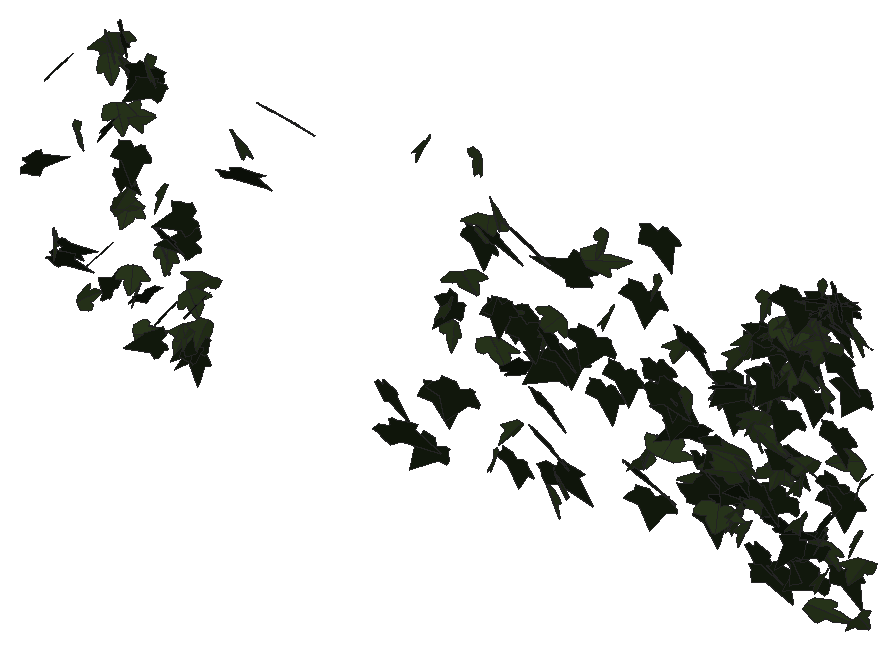
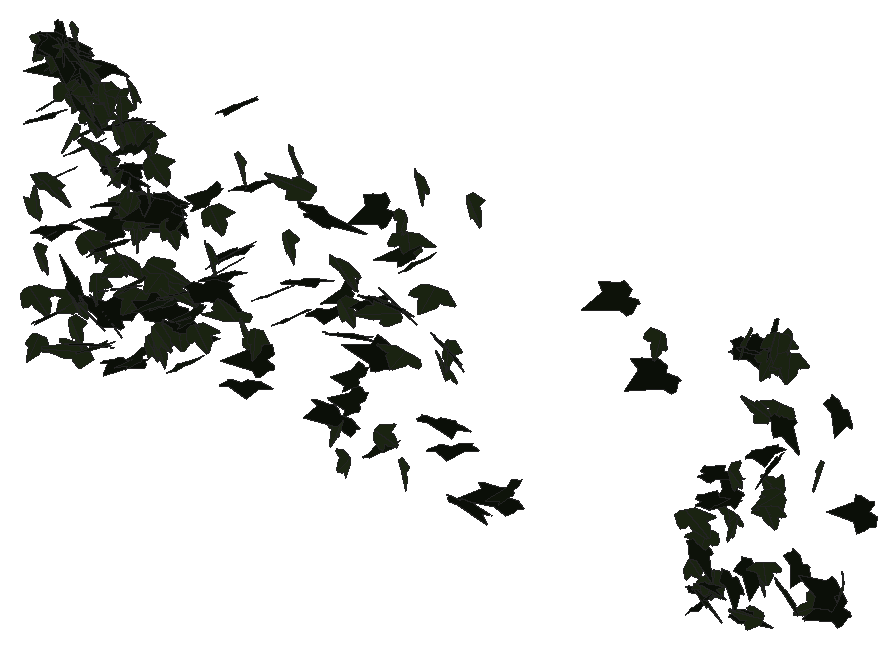
# SketchUp Ruby script. Lengths in millimetres.
U = 1.mm
M = Sketchup.active_model
def pt(a) = Geom::Point3d.new(a.map { |v| v * U })
def face(e, loops, mat)
  f = e.add_face(loops[0].map { |a| pt(a) })
  loops[1..].each { |l| e.add_face(l.map { |a| pt(a) }).erase! }
  f.material = f.back_material = mat if mat
  f
end
# faces: each face lists its corners as indices into pts; further lists are holes
def faces(e, pts, list, mat = nil) = list.each { |f| face(e, (f[0].is_a?(Array) ? f : [f]).map { |l| l.map { |i| pts[i] } }, mat) }
# xy, xz, yz: faces in a plane at the given z, y or x. An outline is a flat list of corners, or four numbers for a rectangle; further outlines are holes
def ring(l) = l.size == 4 ? [[l[0], l[1]], [l[2], l[1]], [l[2], l[3]], [l[0], l[3]]] : l.each_slice(2).to_a
def flat(e, list, mat, &to3) = list.each { |f| face(e, (f[0].is_a?(Array) ? f : [f]).map { |l| ring(l).map { |u, v| to3.(u, v) } }, mat) }
def xy(e, z, list, mat = nil) = flat(e, list, mat) { |x, y| [x, y, z] }
def xz(e, y, list, mat = nil) = flat(e, list, mat) { |x, z| [x, y, z] }
def yz(e, x, list, mat = nil) = flat(e, list, mat) { |y, z| [x, y, z] }
def lines(e, pts, list) = list.each { |a, b| e.add_line(pt(pts[a]), pt(pts[b])) }
# prism: a flat outline (further loops are holes) pulled along v
def prism(e, loops, v, mat = nil)
  f = face(e, loops, mat); d = Geom::Vector3d.new(v.map { |x| x * U })
  f.pushpull(f.normal.samedirection?(d) ? d.length : -d.length)
end
def box(e, o, s, mat = nil) = prism(e, [[o, [o[0] + s[0], o[1], o[2]], [o[0] + s[0], o[1] + s[1], o[2]], [o[0], o[1] + s[1], o[2]]]], [0, 0, s[2]], mat)
def at(x, y, z, deg = 0) = Geom::Transformation.translation(pt([x, y, z])) * Geom::Transformation.rotation(ORIGIN, Z_AXIS, deg.degrees)
def axes(o, x, y, z) = Geom::Transformation.new([*x, 0, *y, 0, *z, 0, *pt(o).to_a, 1])
def part(name) = M.definitions.add(name)
# library, detail: a bought-in or finely detailed component or shape, given as its bounding box
def library(name, o, s) = part(name).tap { |d| box(d.entities, o, s) }
def detail(e, o, s) = box(e.add_group.entities, o, s)
def put(e, d, t, mat = nil) = e.add_instance(d, t).tap { |i| i.material = mat if mat }
def group(e, t, mat = nil) = e.add_group.tap { |g| g.transformation = t; g.material = mat if mat }.entities
root = M.entities
M.materials.add("efeu1").color = [18, 25, 13]
M.materials.add("efeu2").color = [43, 57, 29]
c1 = part("ivyleaf_9")
p = [[39.1,54.8,31.7],[34.5,51.8,30.2],[-5.3,25.2,17.3],[-17.9,28.3,20.9],[-21.6,21.7,17],[-20.2,4.3,5.3],
  [-22.9,-0.3,2.5],[-17.1,-4,-0.6],[-2,-2.1,-1.2],[-0.7,-15.4,-10.1],[16.6,-22.3,-16.7],[21.1,-15.1,-12.5],
  [32.7,-10.7,-11],[46.1,-1.8,-6.6],[30.8,11.2,3.8]]
faces(c1.entities,p,[[0,1,2,3,4,5,6,7,8,9,10,11,12,13,14]],"efeu1")
c2 = part("ivyleaf_10")
p = [[0,12.8,-0.8],[-1.5,51.3,-10.9],[-4.9,51,-11.6],[-13.6,26.5,-7.3],[-13.2,15.9,-4.6],[-21.1,19.3,-7.2],
  [-29.5,16.3,-8.3],[-29.2,8.3,-6.2],[-19.7,-9.8,0.5],[-7.6,-13,4],[1,-12.2,5.8],[-0.4,51.1,-11.1],
  [-1.5,51.1,-10.9],[1,-12.4,5.9],[16.9,-12.4,3.5],[35.1,9.1,-5.1],[35,12.9,-6.1],[20.5,16.4,-4.9],
  [15.8,15,-3.8],[15.3,27.6,-7.1],[12.8,31.3,-7.8]]
faces(c2.entities,p,[[0,1,2,3,4,5,6,7,8,9,10],[11,12,0,13,14,15,16,17,18,19,20]],"efeu2")
put(root,c1,axes([356.5,756.3,2993.2],[0.34233,0.69768,-0.91695],[0.14407,0.92137,0.73718],[1.39828,-0.26574,0.14853]))
put(root,c1,axes([418.9,777,3252.7],[0.1319,0.98378,0.6336],[-0.03652,0.63842,-0.98615],[-1.42713,0.07459,0.08379]))
put(root,c2,axes([403.1,793,2800.9],[-0.36307,0.76759,-0.76025],[0.21719,-0.74294,-0.8198],[-1.30002,-0.3385,0.07536]))
put(root,c1,axes([401.6,799.6,2740.1],[1.21232,0.1716,0.53653],[0.65202,0.05658,-1.00794],[-0.21716,1.12788,-0.03107]))
put(root,c1,axes([421.4,807.3,2769.8],[0.95036,0.3908,-0.68763],[0.74884,0.30998,0.87151],[0.60854,-0.99175,0.00144]))
put(root,c2,axes([458.5,805,3095.3],[-0.68531,0.96396,0.23463],[-0.13774,0.20577,-1.11567],[-1.20251,-0.57293,-0.00592]))
put(root,c2,axes([517.1,757,2684.8],[0.04475,-0.10133,1.11114],[-0.06553,1.11029,0.10303],[-1.35963,-0.05685,0.0316]))
put(root,c1,axes([541.4,772.1,2796.8],[0.26817,0.86274,0.67767],[0.00973,0.68986,-0.88085],[-1.33838,0.17788,0.12938]))
put(root,c2,axes([547.8,807.2,3356.1],[-1.01402,-0.78103,-0.11814],[0.07767,0.1047,-1.14008],[0.96056,-0.83297,-0.03253]))
put(root,c1,axes([578.3,789.1,2721.7],[-0.43352,0.78424,0.68069],[-0.43135,0.58508,-0.85866],[-1.19121,-0.49727,0.06321]))
put(root,c1,axes([585.2,789.4,3174],[-0.53232,0.98978,-0.4697],[0.20509,-0.43911,-1.08148],[-1.32078,-0.4671,0.02137]))
put(root,c2,axes([571.2,780.6,3389.5],[-0.88104,0.89475,-0.19022],[0.1387,-0.15268,-1.1498],[-1.10734,-0.73102,0.00732]))
put(root,c2,axes([569.7,785.1,3330.9],[0.51505,1.08872,0.04324],[0.02313,0.03903,-1.1677],[-1.32908,0.42258,-0.00356]))
put(root,c2,axes([585.9,802,3391.7],[-1.06774,-0.75615,-0.11022],[0.10725,0.06683,-1.15658],[0.92606,-0.87957,0.00687]))
put(root,c1,axes([607.2,784.1,3414],[0.6622,-0.12279,-1.03457],[-1.13242,0.47276,-0.5431],[0.5772,1.06839,0.12142]))
put(root,c2,axes([590.6,788.3,3204.1],[1.27648,0.36666,0.39342],[0.45387,0.128,-1.10868],[-0.47379,1.11046,-0.00211]))
put(root,c2,axes([603.4,815.8,2937.4],[1.23029,0.3806,-0.17497],[-0.19692,-0.06786,-1.07785],[-0.4716,1.02125,-0.00641]))
put(root,c2,axes([602.9,788.6,2962.1],[-0.45813,-0.38786,-0.98717],[0.83705,0.70976,-0.53986],[0.98676,-0.78215,-0.00037]))
put(root,c1,axes([608.7,781.9,3053.1],[0.68449,-0.6018,-0.76512],[-0.51748,0.64372,-0.81735],[1.06892,0.697,0.09426]))
put(root,c2,axes([612.2,777.4,2965.3],[-0.0764,-1.05409,0.53907],[0.03605,0.53827,1.05595],[-1.44396,0.06921,-0.00216]))
put(root,c2,axes([615.8,796.3,3326.9],[-1.3192,0.40401,-0.15754],[0.19032,-0.03247,-1.15407],[-0.49362,-1.09224,-0.02396]))
put(root,c1,axes([616.8,819.6,3093.1],[-0.47829,-1.05459,-0.21128],[0.08194,0.20043,-1.12508],[1.30961,-0.39769,-0.00677]))
put(root,c2,axes([622.4,804.9,2775.9],[1.06437,0.63682,-0.05341],[-0.04737,-0.03739,-1.08011],[-0.77821,0.87327,-0.0073]))
put(root,c2,axes([646.2,797.6,2743.1],[0.62335,-0.92071,-0.02251],[-0.00867,0.0218,-1.05298],[1.12357,0.51097,0.00436]))
put(root,c2,axes([618.7,815,3187.5],[0.42237,-0.21402,-1.07935],[1.26282,-0.32055,0.39557],[-0.45546,-1.08725,0.09584]))
put(root,c1,axes([682.3,786.3,3343.4],[0.44286,0.56089,-0.98218],[-0.69273,-0.80175,-0.6677],[-1.1934,0.67353,0.02311]))
put(root,c1,axes([675,781,2745.6],[0.29378,1.04941,0.05142],[0.0185,0.04928,-1.07668],[-1.28169,0.24125,-0.00375]))
put(root,c2,axes([654.6,798,2626.2],[0.2891,-0.01851,-1.04724],[1.22337,0.31416,0.22135],[0.36911,-1.02673,0.08661]))
put(root,c1,axes([704.7,805.7,2618.9],[-1.07946,-0.09292,0.56212],[-0.67914,-0.08022,-0.88948],[0.14809,-1.04519,0.01829]))
put(root,c1,axes([703.3,793.1,3312.8],[-1.34136,-0.29734,0.28822],[-0.32088,-0.13016,-1.13763],[0.39021,-1.12914,0.05524]))
put(root,c2,axes([688.7,784.5,3359.6],[-0.54799,1.07798,0.22484],[-0.07593,0.21758,-1.16754],[-1.34129,-0.45273,-0.02577]))
put(root,c2,axes([698.7,829.5,3008.7],[0.37157,-0.90811,0.59404],[0.23973,-0.56064,-0.9578],[1.30199,0.36239,0.00682]))
put(root,c1,axes([727.6,796.1,2699.6],[-0.19934,1.01209,0.32974],[-0.0478,0.32766,-1.02511],[-1.29775,-0.16753,-0.01289]))
put(root,c2,axes([714,805.4,2861.3],[-0.84808,0.83202,-0.14465],[0.10722,-0.11506,-1.08418],[-1.0247,-0.70066,0.00627]))
put(root,c2,axes([734.8,794.1,2873.1],[1.29469,-0.21206,0.17514],[0.21265,-0.02144,-1.08213],[0.25955,1.07536,0.01296]))
put(root,c1,axes([730.2,778.9,2929.1],[1.31564,-0.24368,-0.01207],[-0.01369,0.0051,-1.10558],[0.29734,1.07845,0.0025]))
put(root,c1,axes([786.5,815.6,2971.5],[-0.95963,-0.32714,0.70864],[-0.78504,-0.29759,-0.85163],[0.53891,-1.01603,0.02127]))
put(root,c1,axes([788.6,826.3,2901.2],[-0.81032,-0.21197,0.84357],[-0.92564,-0.3778,-0.69232],[0.51888,-1.00501,0.08234]))
put(root,c2,axes([790.9,798.5,2678.7],[-0.45719,-0.93259,0.60477],[0.00861,-0.6402,-0.98286],[1.35603,-0.31036,0.21014]))
put(root,c2,axes([793,801.8,2682.6],[0.4401,1.09946,-0.18153],[-0.26091,-0.11895,-1.14543],[-1.33423,0.38592,0.16411]))
put(root,c1,axes([810.8,817.9,2661.6],[-1.14636,-0.56298,0.2136],[-0.18719,-0.15895,-1.09393],[0.71036,-0.95041,0.05643]))
put(root,c1,axes([818.4,807,2641.9],[-1.1866,0.57833,-0.25387],[0.25064,-0.15111,-1.13131],[-0.72864,-0.99379,0.02428]))
put(root,c1,axes([820.4,803.7,2760],[-0.47716,1.05139,-0.17096],[0.07305,-0.16014,-1.12178],[-1.29749,-0.39567,-0.00028]))
put(root,c1,axes([805.4,816.6,2620.4],[0.02539,-1.10274,0.10467],[0.00627,-0.10459,-1.10293],[1.35137,0.0212,0.00315]))
put(root,c2,axes([811.1,787.8,2784.9],[0.86052,0.84982,0.3555],[0.0653,0.40917,-1.08434],[-1.12194,0.67562,0.20955]))
put(root,c2,axes([844.5,806.5,2834.1],[-1.20026,-0.63198,0.5214],[-0.66958,-0.38533,-0.89259],[1.40821,-0.72187,0.01999]))
put(root,c2,axes([838.4,805.2,2707.8],[-0.32691,-0.91343,0.63261],[0.28616,-0.68259,-0.88624],[1.325,-0.07794,0.34748]))
put(root,c2,axes([962.7,777.8,3256.1],[-1.52598,0.70772,0.23513],[-0.36821,0.13602,-1.06916],[-1.37073,-0.82442,0.02544]))
put(root,c1,axes([944.5,778.5,3165.3],[1.81078,0.43116,0.29051],[0.51701,0.10427,-1.04445],[-0.84366,0.98932,-0.01653]))
put(root,c1,axes([1035,805.7,3350.7],[2.10136,-0.17355,0.00871],[0.09052,0.24793,-1.08883],[0.31808,1.07596,0.2523]))
put(root,c1,axes([1364.1,818,2723.6],[1.02261,-0.91059,-0.11841],[-0.13079,0.09693,-1.05725],[1.74271,0.5416,-0.00987]))
put(root,c1,axes([1427.6,766.8,2662.3],[0.19495,-0.10547,-1.05394],[1.20963,0.85316,-0.02361],[1.61262,-0.62721,0.14512]))
put(root,c2,axes([1501.6,796.5,3433.2],[0.20888,-1.12799,0.06776],[0.00593,-0.06778,-1.13331],[2.15064,0.10974,-0.00345]))
put(root,c1,axes([1526.5,801.5,2629.8],[-1.88101,-0.15828,-0.18142],[0.35062,-0.00368,-1.00042],[0.29501,-1.00485,0.03224]))
put(root,c1,axes([1544.6,816.4,2776.2],[-0.74938,-0.97676,-0.27931],[0.2327,0.25182,-1.05297],[1.91943,-0.41187,0.01861]))
put(root,c2,axes([1570.3,793.6,3022.3],[-0.07449,-1.06551,-0.32741],[0.33891,0.31742,-1.05431],[2.09421,-0.08927,0.15898]))
put(root,c1,axes([1585.8,803.5,3031.2],[-1.73501,0.32366,-0.47038],[0.83967,-0.16321,-0.96736],[-0.6898,-1.01276,0.00557]))
put(root,c2,axes([1582.2,796.1,2970.6],[1.46973,-0.65183,0.47638],[0.70478,-0.29981,-1.01052],[1.36539,0.85639,0.00882]))
put(root,c1,axes([1607.8,788.9,2812.4],[-1.62348,-0.5552,-0.24044],[0.40141,0.11667,-1.01765],[1.07927,-0.87855,0.01681]))
put(root,c2,axes([1636.8,774,3136.2],[-1.51861,-0.71473,-0.37085],[0.63745,0.18018,-1.0679],[1.39362,-0.86125,0.08435]))
put(root,c2,axes([1655.4,799,3443.6],[1.26617,-0.87205,-0.28529],[0.0453,0.36868,-1.07143],[1.74565,0.62295,0.23473]))
put(root,c1,axes([1650.5,816.6,3224],[-0.16174,-1.04011,0.36056],[0.00257,-0.36173,-1.04317],[2.0951,-0.07985,0.02911]))
put(root,c2,axes([1679.7,810.2,3281.3],[-1.60558,-0.71578,0.12035],[0.15725,-0.27804,-1.07442],[1.37241,-0.80553,0.26391]))
put(root,c1,axes([1665.9,816.1,3251.4],[1.39571,-0.82739,-0.07933],[0.13441,0.16744,-1.09346],[1.5762,0.71837,0.16349]))
put(root,c2,axes([1698.9,806.5,3325.1],[-1.19675,0.92464,-0.04747],[-0.13923,-0.10683,-1.11169],[-1.75658,-0.62149,0.12046]))
put(root,c2,axes([1704.4,802.3,2663],[0.45411,-0.97163,-0.25209],[-0.00326,0.25872,-0.9988],[1.91042,0.2314,0.05822]))
put(root,c2,axes([1698.2,804.1,2961.7],[1.82194,0.21211,0.42187],[0.75357,0.15903,-0.97843],[-0.48966,1.03398,0.06394]))
put(root,c2,axes([1744.1,830.5,2746],[-0.08974,-0.74746,0.72575],[0.02464,-0.72686,-0.74776],[1.98267,-0.0248,0.04214]))
put(root,c1,axes([1734,790.6,3081.1],[-1.24796,-0.2797,-0.82476],[1.65408,-0.27643,-0.59722],[-0.1064,-1.01675,0.38925]))
put(root,c1,axes([1757.9,803.9,3079.5],[-1.32016,-0.67132,-0.50091],[1.14081,0.05642,-0.90568],[1.11347,-0.85375,0.33402]))
put(root,c2,axes([1746.2,792.4,3050.7],[0.62541,0.02903,1.02903],[1.27693,0.81321,-0.2372],[-1.48594,0.71104,0.22926]))
put(root,c1,axes([1770.5,801.2,2676.8],[-0.31006,-0.90011,0.48411],[0.15196,-0.49993,-0.90266],[1.93919,-0.10474,0.14814]))
put(root,c1,axes([1763.8,788.4,2922.6],[0.57252,-0.03966,1.04482],[1.69226,0.58171,-0.23392],[-1.04696,0.91857,0.19325]))
put(root,c1,axes([1780.8,772.2,3307.5],[1.9804,-0.52413,-0.14017],[-0.23277,0.06878,-1.16509],[1.006,1.04771,0.00636]))
put(root,c1,axes([1813.4,787,3057],[-0.26842,-1.05826,-0.18674],[-0.02029,0.18971,-1.06704],[2.04509,-0.13701,-0.0351]))
put(root,c1,axes([1825.2,817.6,2860.1],[0.93652,-0.89724,0.28373],[0.21226,-0.26232,-1.02295],[1.77834,0.50382,-0.02732]))
put(root,c2,axes([1858.5,824.1,3045.5],[0.03896,-1.05918,0.27122],[0.0191,-0.27107,-1.05937],[2.08079,0.02232,0.00464]))
put(root,c1,axes([1877,817.3,2960.9],[-1.72302,-0.4986,0.31147],[-0.23687,-0.3964,-0.9963],[1.09351,-0.87149,0.27497]))
put(root,c2,axes([1867.3,808.7,2624],[-1.01141,0.79284,-0.44341],[0.3057,-0.42361,-0.94994],[-1.70165,-0.54734,0.09289]))
put(root,c1,axes([1846,790.8,2775.7],[1.03545,-0.82297,0.36363],[0.36322,-0.30971,-0.98649],[1.67338,0.57646,-0.01088]))
put(root,c2,axes([1907.2,775.4,3117.2],[1.71627,-0.5393,-0.40378],[-0.61592,0.24495,-1.04993],[1.12457,0.9572,0.04119]))
put(root,c1,axes([1874.7,782.2,3059.8],[1.276,-0.87574,-0.1732],[-0.21418,0.13197,-1.10288],[1.68545,0.67977,-0.00902]))
put(root,c2,axes([1915.5,776.6,2690.1],[-1.16386,0.90955,0.26559],[-0.29232,0.21676,-1.096],[-1.77949,-0.63049,0.00634]))
put(root,c1,axes([1912.1,812.8,3009.9],[-0.66778,-0.99722,-0.25343],[0.11587,0.24717,-1.05688],[1.95481,-0.35531,-0.02393]))
put(root,c1,axes([1972.4,802.7,3241.4],[-1.1959,0.24693,0.89941],[-1.60029,0.31932,-0.67511],[-0.76815,-1.04967,0.0062]))
put(root,c1,axes([1910.3,779.3,2715.8],[-0.43449,-0.26158,-1.0719],[1.84713,0.47307,-0.32215],[0.99888,-0.98858,0.12947]))
put(root,c1,axes([1986,824.1,3067.2],[-1.21185,-0.87552,0.14843],[0.06591,-0.20698,-1.07237],[1.68878,-0.62019,0.14836]))
put(root,c2,axes([2034.1,815,3156.5],[0.23589,-1.09728,-0.09636],[-0.00194,0.09685,-1.10421],[2.09638,0.12356,0.00982]))
put(root,c2,axes([2035.1,792.3,3368.6],[1.14713,-0.96262,0.13018],[0.20314,-0.08665,-1.13489],[1.83754,0.61052,0.04419]))
put(root,c2,axes([1997.4,799.9,3293.6],[0.62526,0.0329,-1.08242],[2.03397,0.17281,0.32962],[0.33283,-1.1179,0.0191]))
put(root,c1,axes([2024.4,814.2,2951.7],[-0.11112,-1.07694,0.07568],[-0.00171,-0.07574,-1.07851],[2.05468,-0.05831,0.0032]))
put(root,c1,axes([2069.8,829.1,3006.2],[-0.28255,-1.06241,0.14109],[0.04403,-0.14558,-1.07188],[2.03926,-0.14406,0.04269]))
put(root,c2,axes([2162.5,770.5,2834.4],[-0.30147,-0.92289,-0.52642],[0.16737,0.51902,-0.93638],[2.01515,-0.18117,-0.00098]))
put(root,c1,axes([2152.3,806.1,3256.1],[-0.66408,-1.06136,0.07986],[0.02852,-0.08894,-1.11646],[2.0255,-0.34673,0.04191]))
put(root,c1,axes([2125.5,783.3,2790.8],[1.81332,-0.61478,0.27507],[0.44839,-0.1422,-1.13387],[1.20084,0.98144,0.00802]))
put(root,c1,axes([2176.1,805.6,2719.3],[-1.1359,-0.8177,-0.22652],[0.20845,0.20038,-1.01194],[1.60135,-0.60611,-0.02895]))
put(root,c2,axes([2176.8,784.1,2829.6],[0.95525,-1.01047,0.33531],[-0.28855,0.29908,1.12826],[-2.0056,-0.52431,-0.00262]))
put(root,c2,axes([2194.6,794,3299],[0.60162,-1.03952,-0.31751],[-0.15739,0.3067,-1.08648],[2.06264,0.32661,0.00971]))
put(root,c1,axes([2183.8,806.1,3071.8],[0.358,-1.06563,-0.18462],[0.00775,0.18809,-1.0815],[2.0583,0.18464,0.03618]))
put(root,c1,axes([2204.1,784.8,3442.8],[0.00005,-1.13828,-0.18638],[-0.0161,0.18637,-1.13825],[2.19517,0.00139,-0.00835]))
put(root,c1,axes([2217.5,823.2,3015.8],[-0.21312,-1.02799,0.34018],[-0.11287,-0.33566,-1.03385],[2.05772,-0.12488,-0.02147]))
put(root,c1,axes([2218.2,774.7,3044.8],[0.49939,-0.86938,-0.67513],[-0.09196,0.68428,-0.89994],[2.0929,0.23751,0.12155]))
put(root,c2,axes([2224.4,783.7,2868.4],[1.92224,0.43056,-0.45145],[0.63207,0.35614,1.08267],[1.00509,-1.04742,0.18255]))
put(root,c2,axes([2252.5,818.3,3151.6],[-0.66618,-1.00823,0.27449],[-0.00438,-0.28874,-1.06349],[1.9887,-0.33837,0.08961]))
put(root,c1,axes([2246.6,806.7,2980.5],[-0.81768,-0.9869,0.13227],[-0.07319,-0.12751,-1.07625],[1.89365,-0.43107,0.01552]))
put(root,c1,axes([2279.4,810.5,2944.9],[0.11175,0.39433,-1.01387],[-0.47547,-0.98332,-0.39692],[-2.01507,0.25389,0.03743]))
put(root,c2,axes([2286.7,791.1,3030.2],[1.10861,-0.86043,-0.34942],[-0.14032,0.36832,-1.02987],[1.76187,0.57074,0.13784]))
put(root,c2,axes([2304.5,810.1,2815.7],[-0.78077,-0.92186,0.25569],[-0.1343,-0.24829,-1.0084],[1.81576,-0.41476,0.03536]))
put(root,c1,axes([2270.8,811,3179.1],[0.71114,-1.0709,0.30288],[0.2128,-0.28175,-1.13415],[2.10737,0.38983,0.01232]))
put(root,c1,axes([2306.7,823.4,2859.5],[0.72901,-0.99677,0.07006],[0.03111,-0.06877,-1.06779],[1.90147,0.38328,-0.00939]))
put(root,c1,axes([2351.6,787.1,2783.2],[-1.9633,0.08408,0.36527],[0.69313,-0.02808,1.035],[0.16868,1.09398,-0.0015]))
put(root,c1,axes([2332.3,822.7,2719.3],[-0.12181,-0.9947,0.27218],[0.11467,-0.27584,-0.99392],[1.95935,-0.0457,0.07509]))
put(root,c1,axes([2367,833.6,2898.6],[-1.09871,-0.69178,0.56472],[-0.3525,-0.56507,-0.88155],[1.66262,-0.57695,0.18628]))
put(root,c2,axes([2384.8,819.1,3070.3],[-0.33205,-1.06916,0.16961],[-0.00761,-0.17116,-1.08305],[2.06025,-0.17295,0.02333]))
put(root,c2,axes([2419.9,783.1,2885.4],[-0.8828,-0.03418,1.01927],[-1.89259,-0.23328,-0.46037],[0.43064,-1.09529,0.06625]))
put(root,c2,axes([2384.6,778.9,2773.4],[2.02453,0.44099,-0.03659],[-0.07092,-0.00567,-1.1515],[-0.83919,1.06436,0.00903]))
put(root,c2,axes([2442.9,790.4,2929],[0.53162,0.01691,-1.05814],[-1.95512,0.26726,-0.26691],[0.4839,1.06125,0.08408]))
put(root,c1,axes([2433.6,789.1,3109.4],[0.13878,0.8712,-0.65607],[-0.59379,-0.61339,-0.84921],[-1.9889,0.24392,0.20775]))
put(root,c2,axes([2418.3,812.8,2742],[0.03214,-1.05078,-0.14834],[-0.0552,0.14784,-1.05059],[2.01893,0.02077,-0.02636]))
put(root,c2,axes([2426,807.1,2767.8],[0.08486,-1.02604,0.41002],[-0.00758,-0.4105,-1.02681],[2.10289,0.03993,-0.02025]))
put(root,c1,axes([2422.4,797.5,2834.7],[-0.86454,-0.68394,0.65485],[-0.09311,-0.70839,-0.77379],[1.79971,-0.36519,0.27454]))
put(root,c1,axes([2442.9,796,3119.3],[-1.87088,-0.46707,0.08796],[-0.1442,-0.04549,-1.0883],[0.89299,-0.98589,0.00854]))
put(root,c1,axes([2419.7,809.3,3060.1],[-0.67816,-1.0252,0.15593],[0.01135,-0.1669,-1.08371],[1.97356,-0.35132,0.05981]))
put(root,c1,axes([2396.3,802.2,3096.5],[1.95232,0.09267,0.36656],[0.65117,0.22356,-1.014],[-0.30625,1.06615,0.18076]))
put(root,c1,axes([2423.2,784.7,2803.3],[1.80162,0.32897,0.50604],[-0.90227,-0.17731,1.0021],[0.71096,-1.05865,-0.01059]))
put(root,c2,axes([2447.1,796.6,3205],[-0.55659,-0.99715,0.41347],[-0.18146,-0.40284,-1.03895],[2.04642,-0.30693,0.02033]))
put(root,c2,axes([2435.6,796.4,2908.4],[-1.69659,0.54624,-0.16724],[0.29457,-0.06743,-1.04523],[-1.04658,-0.90448,-0.02308]))
put(root,c1,axes([2431.9,830.7,2841.3],[-0.5742,-0.87595,0.49937],[0.14421,-0.53947,-0.90051],[1.91356,-0.22219,0.21771]))
put(root,c2,axes([2445.3,811,2735.4],[0.05642,-0.97597,0.35183],[0.20262,-0.34725,-0.97224],[1.96405,0.06386,0.09019]))
put(root,c2,axes([2441.4,824.3,3113.6],[-0.07356,0.37648,-1.02131],[0.18465,-1.0167,-0.37845],[-2.06337,-0.10441,0.00254]))
put(root,c2,axes([2485.3,778.5,3266.5],[-0.46484,-1.11085,0.02732],[-0.00992,-0.02683,-1.13738],[2.11478,-0.2443,0.00067]))
put(root,c2,axes([2485.1,794.3,3036],[-1.13709,-0.85008,-0.28649],[0.46109,0.17852,-1.03494],[1.64383,-0.6381,0.09212]))
put(root,c2,axes([2488.2,793.5,3036.1],[-0.16731,-0.92592,-0.55194],[0.29681,0.53702,-0.92574],[2.02996,-0.15484,0.08987]))
put(root,c2,axes([2505.7,782.8,3004.3],[-0.36972,0.49194,0.97774],[-1.11437,0.79228,-0.51496],[-1.75997,-0.60499,0.12066]))
put(root,c1,axes([2469.2,801.4,3256.8],[1.50006,-0.69825,-0.40956],[-0.21327,0.47202,-1.02038],[1.52582,0.75244,0.26003]))
put(root,c1,axes([2475.5,809.5,2685.2],[0.95787,-0.9154,-0.19086],[-0.08214,0.19378,-1.0432],[1.77775,0.50218,0.05464]))
put(root,c2,axes([2510.9,787.5,3065],[-1.20326,-0.86868,0.12919],[-0.09859,-0.12202,-1.07398],[1.66854,-0.63365,0.0297]))
put(root,c2,axes([2496.5,814.2,3108.8],[0.98466,0.95064,0.01218],[-0.05742,0.03027,-1.08153],[-1.80849,0.51663,0.04097]))
put(root,c2,axes([2503.5,785.1,2829.3],[-1.56613,-0.52091,-0.42514],[0.66243,0.24487,-0.97372],[1.09487,-0.89327,-0.019]))
put(root,c2,axes([2508.5,820,3129.6],[-0.08948,0.96333,-0.52592],[-0.10621,-0.52782,-0.96182],[-2.08614,-0.01445,0.07152]))
put(root,c2,axes([2518,791.8,3272.7],[-0.04723,-1.09835,0.21788],[0.02942,-0.21825,-1.09845],[2.13091,-0.02133,0.02]))
put(root,c1,axes([2503.4,797.4,2862.3],[0.335,-1.06453,0.05599],[0.03009,-0.05413,-1.07896],[2.02859,0.1766,0.00676]))
put(root,c1,axes([2541,815.4,3156.7],[-2.04038,-0.20445,-0.16315],[0.3009,0.04185,-1.09134],[0.39659,-1.08361,-0.01137]))
put(root,c2,axes([2527,783.2,3380],[1.28573,-0.89557,0.08296],[0.24472,-0.00652,-1.11747],[1.69416,0.68061,0.09845]))
put(root,c1,axes([2541.7,804.1,3163.2],[-1.24874,-0.85463,0.24147],[-0.31812,-0.17602,-1.07716],[1.66,-0.67663,-0.02478]))
put(root,c1,axes([2538.5,797.9,3276.2],[-1.31162,-0.75384,0.48854],[-0.09844,-0.58142,-0.97013],[1.70681,-0.61283,0.31947]))
put(root,c2,axes([2529.5,817.2,3162.3],[-0.09176,1.05706,-0.31387],[-0.03118,-0.31482,-1.05775],[-2.09838,-0.04155,0.02944]))
put(root,c2,axes([2509.9,780.8,3023.3],[-1.36956,0.13681,-0.83108],[1.4605,-0.34405,-0.7211],[-0.66071,-1.04411,0.12872]))
put(root,c2,axes([2526.7,805.6,2917.4],[-1.3185,-0.5214,-0.62357],[1.05402,0.29695,-0.86357],[1.13236,-0.88352,0.07775]))
put(root,c1,axes([2524.1,801.2,2654.4],[-0.22467,-0.83839,-0.60739],[0.36791,0.58272,-0.84192],[1.93571,-0.20806,0.08952]))
put(root,c1,axes([2549.3,822.2,2845.3],[-1.22794,-0.70565,0.47163],[-0.23274,-0.50895,-0.9288],[1.59849,-0.61618,0.22706]))
put(root,c2,axes([2549.9,803.5,3263.6],[0.27907,-1.11354,0.04185],[-0.00164,-0.04233,-1.12314],[2.12079,0.14649,-0.00637]))
put(root,c2,axes([2542.9,803,2926],[1.40959,-0.75181,0.17822],[0.22371,-0.13437,-1.05531],[1.45339,0.74984,-0.01042]))
put(root,c2,axes([2554.4,779.5,3318.6],[0.03521,-1.07942,-0.36029],[0.13272,0.36074,-1.07717],[2.1617,-0.00457,0.072]))
put(root,c2,axes([2556.5,821.2,3177.2],[0.46043,-1.06671,0.1041],[0.00152,-0.10654,-1.09357],[2.03981,0.24086,-0.02268]))
put(root,c1,axes([2547.5,797.7,3275.9],[-0.57126,-1.07769,0.07527],[-0.02161,-0.07497,-1.11867],[2.05595,-0.30023,0.00916]))
put(root,c1,axes([2557.8,821.6,3074],[-0.81787,-0.96127,0.22537],[-0.04679,-0.2353,-1.05049],[1.87852,-0.42438,0.07196]))
put(root,c1,axes([2549.9,816.3,2964.2],[0.34928,-0.95892,-0.49518],[0.11702,0.51076,-0.96631],[2.05065,0.13418,0.13949]))
put(root,c1,axes([2539.8,809.3,2766.3],[0.71227,-0.36626,0.9382],[1.67002,-0.37272,-0.49553],[0.94089,0.93881,0.1693]))
put(root,c1,axes([2547.9,794.6,2999.3],[1.28827,-0.73553,0.41424],[0.66342,-0.24005,-0.99582],[1.46323,0.75641,0.08679]))
put(root,c2,axes([2576.4,771.3,3336.1],[0.66399,1.06413,0.14299],[0.11919,0.12992,-1.1197],[-2.03998,0.35395,-0.01888]))
put(root,c2,axes([2592.6,791.4,3348.6],[-0.2117,-1.11497,-0.16054],[0.03866,0.1593,-1.12049],[2.14354,-0.11299,0.00435]))
put(root,c1,axes([2613.8,791.8,2763.3],[-1.76212,0.45968,-0.57096],[0.98738,-0.23886,-1.0336],[-0.98553,-1.06121,-0.01468]))
put(root,c1,axes([2605.5,837.2,2671],[-0.92503,-0.67717,0.61335],[-0.18677,-0.65202,-0.79763],[1.7288,-0.43277,0.24201]))
put(root,c2,axes([2618.4,827.9,2957],[-0.658,-0.81918,0.59777],[-0.22957,-0.59385,-0.88358],[1.91633,-0.35242,0.09941]))
put(root,c2,axes([2608.2,813,3201.3],[1.99023,-0.33669,-0.15025],[-0.27004,0.04957,-1.09859],[0.64765,1.0553,0.00366]))
put(root,c1,axes([2593.9,795.7,3279.6],[-0.16597,-1.08107,0.25852],[0.05034,-0.26126,-1.0836],[2.1149,-0.07862,0.04608]))
put(root,c2,axes([2622.2,798.5,3281.8],[-1.04485,-0.9803,0.01438],[0.02388,-0.0235,-1.12333],[1.86575,-0.54868,0.02243]))
put(root,c2,axes([2624.1,784.9,2825.9],[-0.26,-1.01579,-0.30349],[0.14136,0.29608,-1.02442],[2.01274,-0.15201,0.03274]))
put(root,c2,axes([2625.6,802.2,3344.2],[1.26024,0.8138,-0.41376],[-0.47597,-0.32989,-1.04908],[-1.67105,0.7077,-0.01323]))
put(root,c2,axes([2628.2,774.9,2932.8],[0.00405,-1.00701,-0.39543],[0.2118,0.39354,-1.00159],[2.04809,-0.0387,0.10436]))
put(root,c1,axes([2624.6,792.2,3411.5],[-1.64292,-0.58963,-0.44642],[0.8195,0.15716,-1.04021],[1.14437,-0.95905,0.104]))
put(root,c1,axes([2606.7,820.3,3251.4],[0.47954,-1.06277,-0.14593],[0.03784,0.1545,-1.09087],[2.0413,0.2468,0.0545]))
put(root,c1,axes([2644,823.1,2666.6],[-1.60062,-0.46078,0.40771],[-0.33856,-0.47892,-0.90821],[1.12095,-0.8026,0.30786]))
put(root,c2,axes([2634.9,805.4,3307.3],[0.67604,-1.05413,0.15556],[0.07767,-0.1504,-1.11233],[2.02646,0.35743,-0.00926]))
put(root,c1,axes([2651.4,798.5,3382.5],[-1.16894,0.4812,-0.81978],[1.06899,-0.60368,-0.77518],[-1.45952,-0.82755,0.0888]))
put(root,c1,axes([2666.7,799.3,3312.1],[-0.98161,0.9728,-0.16272],[0.19563,-0.12961,-1.10066],[-1.86692,-0.52507,-0.02978]))
put(root,c2,axes([2638.8,798.3,3343.5],[-1.40443,-0.66183,-0.54507],[0.79715,0.34924,-0.99109],[1.42384,-0.84834,0.01723]))
put(root,c2,axes([2682.9,795.8,3387.9],[-1.47128,-0.28997,0.77562],[-1.26205,-0.4187,-0.81746],[0.94383,-1.01187,0.11599]))
put(root,c1,axes([2676.2,806.3,2769.8],[-1.69434,0.53258,-0.22377],[0.34672,-0.13129,-1.03724],[-1.04335,-0.90852,0.01871]))
put(root,c2,axes([2665.8,822.1,2786.5],[0.75834,-0.93808,0.28861],[0.14477,-0.28103,-1.01847],[1.86232,0.40383,-0.03835]))
put(root,c1,axes([2659.9,794.7,3168.3],[-0.42783,-1.03025,0.37247],[0.06278,-0.38642,-1.04893],[2.08403,-0.19986,0.10806]))
put(root,c2,axes([2669.2,784.5,3318.1],[-0.81999,-0.9586,-0.40807],[0.53573,0.31806,-1.04436],[1.9091,-0.50099,0.11779]))
put(root,c1,axes([2658.6,815.6,2797.1],[0.26801,0.85675,0.68004],[-0.27768,-0.66481,0.86778],[2.06319,-0.20077,0.02845]))
put(root,c2,axes([2684.5,795.8,2693.8],[0.13055,-1.06761,0.04154],[-0.00683,-0.04186,-1.06979],[2.03339,0.0684,-0.00626]))
put(root,c2,axes([2679.7,792.5,3408.5],[1.34919,-0.88264,0.03321],[0.02031,-0.03402,-1.13201],[1.68091,0.70887,-0.01298]))
put(root,c2,axes([2675.2,800.6,3347.6],[-0.42171,1.08904,-0.20861],[0.12148,-0.19986,-1.11113],[-2.10685,-0.22951,-0.02231]))
put(root,c2,axes([2674.1,807.3,2766.5],[-1.73862,0.30764,-0.44243],[0.71384,-0.26225,-0.9568],[-0.7364,-0.98056,0.11709]))
put(root,c1,axes([2714.4,785.3,3425.3],[-1.28846,0.90377,-0.17907],[0.07638,-0.19307,-1.12619],[-1.75182,-0.67314,0.0826]))
put(root,c2,axes([2693,785.6,3464.7],[0.82031,-1.05959,-0.14282],[0.03271,0.16084,-1.14137],[2.03458,0.42462,0.07594]))
put(root,c2,axes([2704.6,791.1,3312.9],[-1.21063,-0.8307,0.41785],[-0.28167,-0.40937,-1.03913],[1.74717,-0.64159,0.12201]))
put(root,c1,axes([2717.1,794.6,3427.7],[0.9199,0.75974,-0.69885],[-0.91385,-0.51763,-0.89483],[-1.73916,0.67385,0.10055]))
put(root,c2,axes([2695.7,780.7,3199.5],[0.92527,-0.72671,-0.71756],[0.45379,0.85352,-0.70286],[1.88997,0.15084,0.52005]))
put(root,c1,axes([2711.7,792.5,3419.1],[0.55716,1.10256,0.05759],[-0.02283,0.06275,-1.14043],[-2.10114,0.29169,0.02766]))
put(root,c2,axes([2712.5,792.8,3423],[-0.42688,1.09547,0.15556],[-0.32355,0.12272,-1.10932],[-2.0808,-0.24382,0.14058]))
put(root,c2,axes([2679,779.1,2615],[-0.67221,-0.13813,-1.03534],[1.96604,0.11553,-0.36782],[0.29416,-1.08781,0.09241]))
put(root,c1,axes([2736.7,782.7,3458],[0.64524,-0.18207,-1.08033],[-1.8964,0.41884,-0.38329],[0.86674,1.05196,-0.03437]))
put(root,c2,axes([2711.7,794.3,3409.5],[0.94118,0.88418,0.52386],[0.04324,0.5718,-0.98655],[-1.95547,0.43821,0.23032]))
put(root,c1,axes([2686.2,798.4,3378.1],[1.85985,-0.56405,0.10988],[0.44783,0.195,-1.0917],[0.99779,0.96385,0.28516]))
put(root,c1,axes([2717.7,810.7,2938.9],[-0.38355,-0.96439,0.4365],[-0.12509,-0.43208,-0.98498],[2.0108,-0.21083,0.02198]))
put(root,c1,axes([2706.4,795,3438.5],[-0.95461,-0.50398,-0.88565],[1.20615,0.61871,-0.711],[1.51868,-0.80818,0.00798]))
put(root,c1,axes([2717.9,810.7,3083.5],[-0.04039,-1.08647,0.13075],[0.0294,-0.13106,-1.08653],[2.08248,-0.01922,0.01787]))
put(root,c1,axes([2713.9,799.6,3391.9],[0.47235,-1.10286,-0.01708],[-0.03239,0.01368,-1.13036],[2.09897,0.2484,-0.0136]))
put(root,c1,axes([2721.8,801.5,3285.5],[0.60001,-1.03402,-0.27569],[-0.14786,0.26453,-1.08101],[2.03132,0.32468,0.00275]))
put(root,c1,axes([2733.2,816.7,2711.9],[0.21221,-1.04762,-0.20298],[-0.02896,0.2025,-1.05352],[2.0307,0.11237,0.00618]))
put(root,c1,axes([2746.2,794.7,2928.8],[-0.70461,-0.98904,-0.18845],[0.08776,0.18392,-1.05585],[1.91419,-0.3725,-0.02096]))
put(root,c2,axes([2783.5,784.9,3038.7],[1.32134,-0.37417,-0.80668],[-1.38159,0.35259,-0.78832],[0.97743,1.0042,-0.02378]))
put(root,c2,axes([2786.3,818,2749],[-0.96022,-0.91681,0.45278],[-0.19267,-0.45763,-1.03944],[1.93651,-0.50014,0.1211]))
put(root,c1,axes([2776.3,808.1,3216.6],[-0.84589,-0.91237,0.45193],[-0.25663,-0.43602,-1.01287],[1.9207,-0.46007,0.0637]))
put(root,c2,axes([2788.7,799.7,2615.1],[-0.51181,-0.79208,-0.61992],[0.44774,0.57436,-0.83592],[1.86119,-0.35598,0.03062]))
put(root,c2,axes([2787.8,775.6,3394.4],[-1.43113,0.84847,-0.21901],[0.25954,-0.17177,-1.13367],[-1.64741,-0.76413,0.01166]))
put(root,c2,axes([2795.2,787.7,2839.2],[0.5376,-1.005,0.27621],[0.14302,-0.26579,-1.04394],[1.97847,0.2923,0.00041]))
put(root,c2,axes([2788.5,809.8,2963.6],[-0.14846,-0.79421,-0.75869],[0.13577,-0.76265,0.79103],[-2.08596,0.00689,0.10548]))
